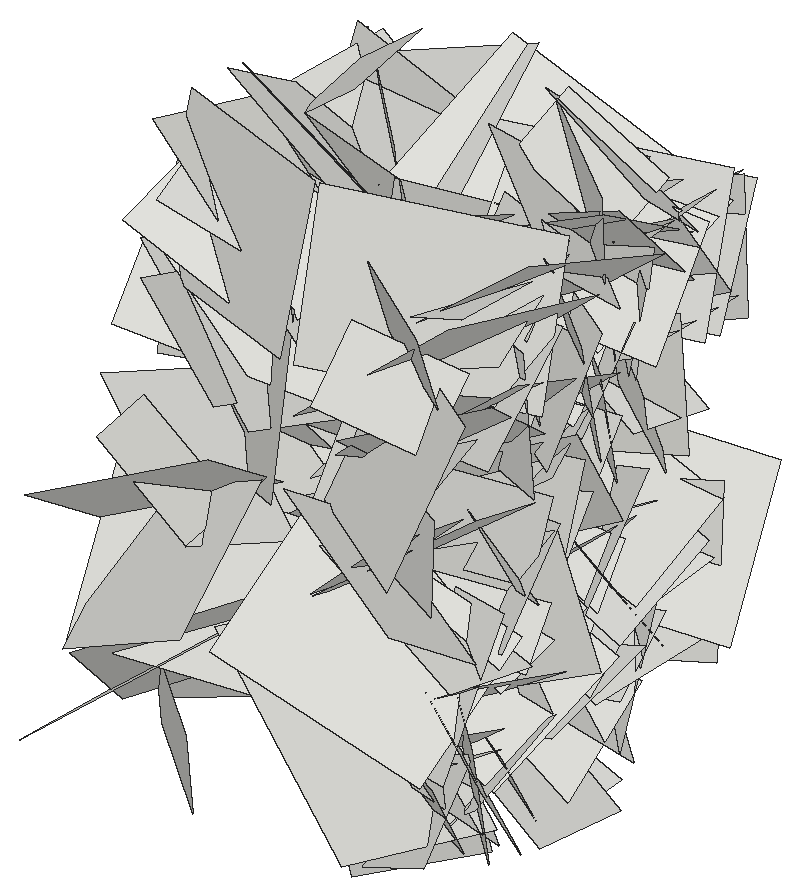
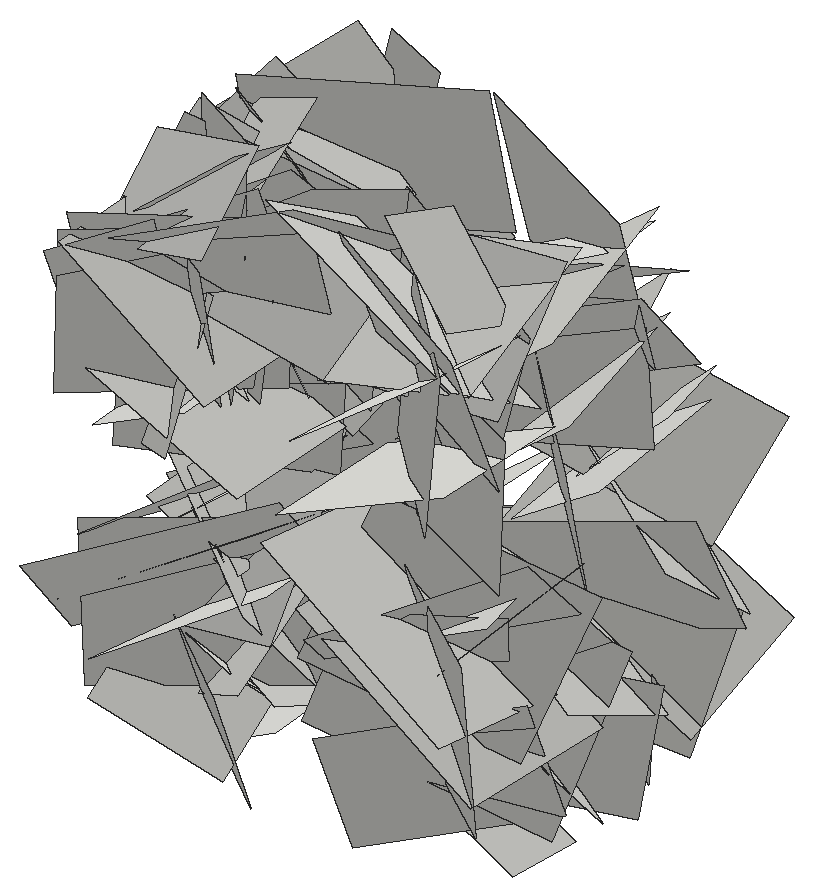
# SketchUp Ruby script. Lengths in inches.
U = 1.inch
M = Sketchup.active_model
def pt(a) = Geom::Point3d.new(a.map { |v| v * U })
def face(e, loops, mat)
  f = e.add_face(loops[0].map { |a| pt(a) })
  loops[1..].each { |l| e.add_face(l.map { |a| pt(a) }).erase! }
  f.material = f.back_material = mat if mat
  f
end
# faces: each face lists its corners as indices into pts; further lists are holes
def faces(e, pts, list, mat = nil) = list.each { |f| face(e, (f[0].is_a?(Array) ? f : [f]).map { |l| l.map { |i| pts[i] } }, mat) }
# xy, xz, yz: faces in a plane at the given z, y or x. An outline is a flat list of corners, or four numbers for a rectangle; further outlines are holes
def ring(l) = l.size == 4 ? [[l[0], l[1]], [l[2], l[1]], [l[2], l[3]], [l[0], l[3]]] : l.each_slice(2).to_a
def flat(e, list, mat, &to3) = list.each { |f| face(e, (f[0].is_a?(Array) ? f : [f]).map { |l| ring(l).map { |u, v| to3.(u, v) } }, mat) }
def xy(e, z, list, mat = nil) = flat(e, list, mat) { |x, y| [x, y, z] }
def xz(e, y, list, mat = nil) = flat(e, list, mat) { |x, z| [x, y, z] }
def yz(e, x, list, mat = nil) = flat(e, list, mat) { |y, z| [x, y, z] }
def lines(e, pts, list) = list.each { |a, b| e.add_line(pt(pts[a]), pt(pts[b])) }
# prism: a flat outline (further loops are holes) pulled along v
def prism(e, loops, v, mat = nil)
  f = face(e, loops, mat); d = Geom::Vector3d.new(v.map { |x| x * U })
  f.pushpull(f.normal.samedirection?(d) ? d.length : -d.length)
end
def box(e, o, s, mat = nil) = prism(e, [[o, [o[0] + s[0], o[1], o[2]], [o[0] + s[0], o[1] + s[1], o[2]], [o[0], o[1] + s[1], o[2]]]], [0, 0, s[2]], mat)
def at(x, y, z, deg = 0) = Geom::Transformation.translation(pt([x, y, z])) * Geom::Transformation.rotation(ORIGIN, Z_AXIS, deg.degrees)
def axes(o, x, y, z) = Geom::Transformation.new([*x, 0, *y, 0, *z, 0, *pt(o).to_a, 1])
def part(name) = M.definitions.add(name)
# library, detail: a bought-in or finely detailed component or shape, given as its bounding box
def library(name, o, s) = part(name).tap { |d| box(d.entities, o, s) }
def detail(e, o, s) = box(e.add_group.entities, o, s)
def put(e, d, t, mat = nil) = e.add_instance(d, t).tap { |i| i.material = mat if mat }
def group(e, t, mat = nil) = e.add_group.tap { |g| g.transformation = t; g.material = mat if mat }.entities
root = M.entities
c1 = part("Component\#6")
p = [[0.01,0,0],[0,3.24,4.54],[4.32,3.24,4.54],[4.33,0,0]]
faces(c1.entities,p,[[0,1,2,3]])
put(root,c1,axes([400.91,173.53,27.66],[0.08068,-0.97468,-0.75893],[0.01331,-0.75972,0.97695],[1.30935,0.06778,0.03684]))
put(root,c1,axes([414.68,173.53,27.66],[-0.08068,-0.97468,-0.75893],[-0.01331,-0.75972,0.97695],[-1.30935,0.06778,0.03684]))
put(root,c1,axes([400.91,172.42,21.79],[0.22827,-1.35966,0.24048],[-0.1567,0.21929,1.3722],[1.45519,0.2369,0.11004]))
put(root,c1,axes([414.68,172.42,21.79],[-0.22827,-1.35966,0.24048],[0.1567,0.21929,1.3722],[-1.45519,0.2369,0.11004]))
put(root,c1,axes([410.71,168.82,35.84],[0.04533,0.37689,0.51175],[-0.01637,0.51337,-0.3768],[0.67349,-0.01289,-0.04361]))
put(root,c1,axes([400.91,171.44,27.64],[0.05126,-0.8571,0.56567],[0.11133,0.56746,0.85083],[1.08285,-0.01777,-0.11425]))
put(root,c1,axes([414.68,171.44,27.64],[-0.05126,-0.8571,0.56567],[-0.11133,0.56746,0.85083],[-1.08285,-0.01777,-0.11425]))
put(root,c1,axes([414.68,167.34,31.77],[0.2501,0.51374,1.1242],[0.05799,1.13903,-0.532],[-1.3089,0.14863,0.19123]))
put(root,c1,axes([410.71,172.01,32.68],[0.01531,-0.04852,-0.71126],[0.05574,-0.70939,0.04946],[0.75363,0.05345,0.01079]))
put(root,c1,axes([404.88,172.58,29],[0.14706,-0.68518,0.03236],[0.10474,0.05263,0.69082],[-0.71951,-0.13238,0.10718]))
put(root,c1,axes([410.71,172.58,29],[-0.14706,-0.68518,0.03236],[-0.10474,0.05263,0.69082],[0.71951,-0.13238,0.10718]))
put(root,c1,axes([410.71,170.91,25.11],[0.00896,0.33986,-0.6335],[0.15678,-0.62081,-0.33108],[0.74574,0.12644,0.07722]))
put(root,c1,axes([410.71,171.42,39.46],[0.01769,0.21401,-0.61924],[0.03571,-0.6189,-0.21298],[0.69357,0.02641,0.02676]))
put(root,c1,axes([414.68,169.05,21.98],[-0.04882,0.58162,0.59704],[0.02934,0.59868,-0.58109],[-0.88303,-0.01226,-0.05232]))
put(root,c1,axes([410.71,173.67,32.24],[-0.05341,-0.65994,-0.37026],[-0.06447,-0.36634,0.66124],[0.79951,-0.07362,0.02859]))
put(root,c1,axes([404.88,170.73,19.61],[0.06378,-0.15247,0.68566],[0.07422,0.68605,0.14641],[-0.74085,0.05561,0.0737]))
put(root,c1,axes([410.71,170.73,19.61],[-0.06378,-0.15247,0.68566],[-0.07422,0.68605,0.14641],[0.74085,0.05561,0.0737]))
put(root,c1,axes([410.71,173.11,21.9],[-0.05319,-0.68826,0.19248],[-0.04456,0.19546,0.68797],[0.75624,-0.03689,0.05408]))
put(root,c1,axes([410.71,173.29,20.87],[0.09428,-0.62013,-0.08152],[0.03551,-0.0775,0.6261],[0.66205,0.09247,-0.02197]))
put(root,c1,axes([410.71,173.15,22.23],[0.01199,-0.5915,0.12784],[0.10227,0.12799,0.58366],[0.63327,-0.00947,-0.09668]))
put(root,c1,axes([414.68,174.01,26.46],[0.07872,-0.97306,0.24072],[-0.0738,0.23579,0.97461],[-1.05998,-0.08868,-0.04998]))
put(root,c1,axes([400.91,172.46,21.25],[0.14489,-0.73421,0.72244],[-0.08794,0.71856,0.74596],[1.0883,0.15581,-0.0359]))
put(root,c1,axes([414.68,172.46,21.25],[-0.14489,-0.73421,0.72244],[0.08794,0.71856,0.74596],[-1.0883,0.15581,-0.0359]))
put(root,c1,axes([400.91,169.91,24.28],[-0.0494,0.58776,1.07494],[0.25393,1.05932,-0.56884],[1.27358,-0.18841,0.15511]))
put(root,c1,axes([414.68,169.91,24.28],[0.0494,0.58776,1.07494],[-0.25393,1.05932,-0.56884],[-1.27358,-0.18841,0.15511]))
put(root,c1,axes([404.88,173.74,31.89],[0.15856,-0.67469,0.29232],[0.1064,0.31425,0.67394],[-0.77211,-0.09525,0.1529]))
put(root,c1,axes([410.71,173.74,31.89],[-0.15856,-0.67469,0.29232],[-0.1064,0.31425,0.67394],[0.77211,-0.09525,0.1529]))
put(root,c1,axes([414.68,172.13,35.78],[-0.07615,0.65901,-0.5201],[-0.04859,-0.52431,-0.658],[-0.88857,-0.02781,0.08055]))
put(root,c1,axes([400.91,171.47,32.36],[0.16942,0.96147,-0.31887],[-0.08969,-0.30901,-0.97416],[1.06999,-0.17814,-0.03117]))
put(root,c1,axes([414.68,171.47,32.36],[-0.16942,0.96147,-0.31887],[0.08969,-0.30901,-0.97416],[-1.06999,-0.17814,-0.03117]))
put(root,c1,axes([414.68,173.5,20.5],[0.29119,-0.77592,0.90535],[-0.00734,0.92801,0.79744],[-1.26387,-0.18415,0.20396]))
put(root,c1,axes([414.68,171.18,26.98],[0.09963,0.88743,-0.23237],[-0.05305,-0.22828,-0.89204],[-0.97094,0.10354,0.02489]))
put(root,c1,axes([414.68,170.16,39.2],[0.24703,1.2789,-0.21613],[0.13589,-0.24123,-1.28918],[-1.36812,0.20696,-0.16707]))
put(root,c1,axes([414.68,172,20.82],[0.19013,-0.4174,1.11707],[0.18593,1.12659,0.39279],[-1.25031,0.10406,0.22828]))
put(root,c1,axes([400.91,175.66,39.88],[-0.03914,-0.32872,-1.22009],[0.25418,-1.20026,0.31612],[1.31508,0.2222,-0.09741]))
put(root,c1,axes([414.68,175.66,39.88],[0.03914,-0.32872,-1.22009],[-0.25418,-1.20026,0.31612],[-1.31508,0.2222,-0.09741]))
put(root,c1,axes([410.71,171.52,27.71],[-0.03995,0.48298,0.66079],[-0.01207,0.66111,-0.48387],[0.8675,0.03144,0.0237]))
put(root,c1,axes([414.68,171.36,22.89],[-0.02535,0.88672,0.32576],[0.06435,0.32663,-0.88464],[-0.99927,-0.00146,-0.06523]))
put(root,c1,axes([414.68,175.14,30.45],[0.22771,0.17317,-1.07869],[-0.0194,-1.09862,-0.18001],[-1.15789,0.05246,-0.20912]))
put(root,c1,axes([414.68,174.95,31.63],[-0.12097,-0.07785,-0.70642],[-0.09105,-0.70871,0.09198],[-0.74781,0.09888,0.10307]))
put(root,c1,axes([414.68,176.52,27.27],[-0.06139,-0.83333,-0.30669],[0.14477,-0.31205,0.82208],[-0.93005,0.00643,0.1482]))
put(root,c1,axes([404.88,176.07,37.03],[0.15674,-0.62528,-0.09698],[-0.10666,-0.12156,0.63036],[-0.66219,-0.12843,-0.12449]))
put(root,c1,axes([410.71,176.07,37.03],[-0.15674,-0.62528,-0.09698],[0.10666,-0.12156,0.63036],[0.66219,-0.12843,-0.12449]))
put(root,c1,axes([400.91,172.47,36.95],[0.1233,0.89549,0.4145],[0.21728,0.38634,-0.89217],[1.02316,-0.18996,0.13951]))
put(root,c1,axes([414.68,172.47,36.95],[-0.1233,0.89549,0.4145],[-0.21728,0.38634,-0.89217],[-1.02316,-0.18996,0.13951]))
put(root,c1,axes([414.68,174.16,29.86],[-0.19319,0.59277,-0.26834],[-0.07097,-0.29428,-0.60458],[-0.68606,-0.13648,0.1381]))
put(root,c1,axes([414.68,171.95,33.74],[0.07102,0.70639,0.8167],[-0.11892,0.8184,-0.69866],[-1.13841,-0.04142,0.12393]))
put(root,c1,axes([400.91,171.95,33.74],[-0.07102,0.70639,0.8167],[0.11892,0.8184,-0.69866],[1.13841,-0.04142,0.12393]))
put(root,c1,axes([400.91,177.96,25.04],[0.10915,-1.1796,-0.55067],[0.03689,-0.5497,1.18402],[1.37942,0.10803,0.01191]))
put(root,c1,axes([414.68,177.96,25.04],[-0.10915,-1.1796,-0.55067],[-0.03689,-0.5497,1.18402],[-1.37942,0.10803,0.01191]))
put(root,c1,axes([400.91,178.09,32.9],[0.18757,-0.47698,-1.21124],[-0.23196,-1.21588,0.44684],[1.36024,-0.14157,0.24323]))
put(root,c1,axes([414.68,178.09,32.9],[-0.18757,-0.47698,-1.21124],[0.23196,-1.21588,0.44684],[-1.36024,-0.14157,0.24323]))
put(root,c1,axes([400.91,173.31,35.98],[-0.01252,1.07454,-0.37217],[-0.12805,-0.37127,-1.06811],[1.19858,-0.02844,-0.11799]))
put(root,c1,axes([414.68,173.31,35.98],[0.01252,1.07454,-0.37217],[0.12805,-0.37127,-1.06811],[-1.19858,-0.02844,-0.11799]))
put(root,c1,axes([414.68,176.41,32.2],[-0.11408,-0.0942,-0.79779],[-0.0272,-0.8041,0.09841],[-0.85109,0.03832,0.10379]))
put(root,c1,axes([414.68,172.625,27.43],[0.01975,0.58315,0.74345],[-0.01761,0.74368,-0.58292],[-1.00141,-0.00157,0.02491]))
put(root,c1,axes([400.91,174.78,20.26],[0.10048,-0.39109,0.79293],[0.10042,0.79738,0.38196],[0.93179,-0.04376,-0.12667]))
put(root,c1,axes([414.68,174.78,20.26],[-0.10048,-0.39109,0.79293],[-0.10042,0.79738,0.38196],[-0.93179,-0.04376,-0.12667]))
put(root,c1,axes([410.71,174.375,32.02],[-0.18574,0.64681,-0.5499],[-0.00393,-0.56207,-0.65994],[0.8999,0.13105,-0.11638]))
put(root,c1,axes([400.91,174.06,31.875],[0.08593,-0.00736,1.08266],[0.18405,1.07173,-0.00571],[1.1328,-0.17357,-0.0812]))
put(root,c1,axes([414.68,174.06,31.875],[-0.08593,-0.00736,1.08266],[-0.18405,1.07173,-0.00571],[-1.1328,-0.17357,-0.0812]))
put(root,c1,axes([414.68,176.05,33.17],[-0.01986,0.50916,-0.88553],[0.06176,-0.8837,-0.50934],[-1.08099,-0.05984,-0.01283]))
put(root,c1,axes([414.68,178.05,19.9375],[0.14578,-1.0409,0.22357],[0.02192,0.228,1.04879],[-1.1283,-0.13006,0.04926]))
put(root,c1,axes([410.71,177.7,39.03],[-0.08239,-0.33737,-0.64844],[0.10668,-0.65083,0.32654],[0.76743,0.05425,-0.11501]))
put(root,c1,axes([410.71,173.36,27.66],[-0.12062,0.63946,0.63128],[-0.06443,0.62939,-0.6485],[0.9503,0.12384,0.03616]))
put(root,c1,axes([400.91,173.84,39.64],[-0.13369,1.27699,-0.41872],[-0.11509,-0.42887,-1.27523],[1.41986,0.08547,-0.14279]))
put(root,c1,axes([414.68,173.84,39.64],[0.13369,1.27699,-0.41872],[0.11509,-0.42887,-1.27523],[-1.41986,0.08547,-0.14279]))
put(root,c1,axes([400.91,179.04,23.77],[0.11323,-0.75693,-0.7774],[0.09292,-0.77258,0.76428],[1.14637,0.13739,0.01483]))
put(root,c1,axes([414.68,179.04,23.77],[-0.11323,-0.75693,-0.7774],[-0.09292,-0.77258,0.76428],[-1.14637,0.13739,0.01483]))
put(root,c1,axes([414.68,174.875,32.24],[-0.12053,0.70886,0.38052],[0.08644,0.39248,-0.70676],[-0.84842,-0.06072,-0.12606]))
put(root,c1,axes([410.71,178.15,33.23],[0.08938,-0.00525,-0.60269],[-0.06829,-0.60515,-0.00374],[0.63521,-0.06432,0.0844]))
put(root,c1,axes([414.68,174.67,32.54],[0.17055,0.3665,0.95024],[0.03456,0.95968,-0.37566],[-1.07902,0.08867,0.13816]))
put(root,c1,axes([414.68,174.9,23.69],[0.06803,0.90477,0.33383],[-0.16872,0.33992,-0.89067],[-1.00823,0.00417,0.17157]))
put(root,c1,axes([410.71,175.43,34.87],[-0.0411,0.62613,0.35799],[-0.03637,0.3565,-0.62724],[0.76365,0.05068,-0.01061]))
put(root,c1,axes([414.68,178.01,36.42],[-0.04909,-0.68925,0.58112],[0.09024,0.57594,0.68989],[-0.95135,0.0902,0.03545]))
put(root,c1,axes([404.88,176.44,21.6],[0.04345,0.60879,-0.00304],[-0.10651,0.00376,-0.60183],[-0.63647,0.04093,0.10051]))
put(root,c1,axes([410.71,176.44,21.6],[-0.04345,0.60879,-0.00304],[0.10651,0.00376,-0.60183],[0.63647,0.04093,0.10051]))
put(root,c1,axes([404.88,180.42,25.12],[0.17902,-0.88337,-0.09354],[0.21931,-0.05348,0.8786],[-0.91571,-0.1855,0.19214]))
put(root,c1,axes([410.71,180.42,25.12],[-0.17902,-0.88337,-0.09354],[-0.21931,-0.05348,0.8786],[0.91571,-0.1855,0.19214]))
put(root,c1,axes([414.68,177.13,31.79],[0.078,-0.30439,1.03044],[0.07955,1.03178,0.29943],[-1.13614,0.05135,0.09171]))
put(root,c1,axes([400.91,179.625,37.91],[0.28026,0.12179,-1.29213],[0.26115,-1.29941,-0.07206],[1.35072,0.22596,0.28204]))
put(root,c1,axes([414.68,179.625,37.91],[-0.28026,0.12179,-1.29213],[-0.26115,-1.29941,-0.07206],[-1.35072,0.22596,0.28204]))
put(root,c1,axes([400.91,178.68,21.25],[0.14964,-1.02559,0.91665],[-0.24358,0.89093,1.03221],[1.43757,0.25771,0.07948]))
put(root,c1,axes([414.68,178.68,21.25],[-0.14964,-1.02559,0.91665],[0.24358,0.89093,1.03221],[-1.43757,0.25771,0.07948]))
put(root,c1,axes([414.68,176.26,32.94],[-0.03084,0.60524,0.59943],[0.03406,0.60013,-0.60439],[-0.90231,0.00196,-0.0433]))
put(root,c1,axes([400.91,177.97,39.67],[-0.02985,0.75948,-0.84861],[0.27983,-0.8214,-0.74388],[1.17429,0.21504,0.15569]))
put(root,c1,axes([414.68,177.97,39.67],[0.02985,0.75948,-0.84861],[-0.27983,-0.8214,-0.74388],[-1.17429,0.21504,0.15569]))
put(root,c1,axes([414.68,182.1,27.04],[0.18817,-1.1788,-0.21223],[0.10509,-0.19936,1.19019],[-1.26526,-0.19187,0.06729]))
put(root,c1,axes([400.91,177.28,39.83],[0.04784,1.11638,-0.64936],[0.22797,-0.64718,-1.09769],[1.34988,0.06974,0.20839]))
put(root,c1,axes([414.68,177.28,39.83],[-0.04784,1.11638,-0.64936],[-0.22797,-0.64718,-1.09769],[-1.34988,0.06974,0.20839]))
put(root,c1,axes([410.71,175.72,36.8],[-0.15665,0.75943,0.7145],[-0.11122,0.70715,-0.77331],[1.09966,0.17971,0.02357]))
put(root,c1,axes([410.71,180.11,41],[-0.0874,0.13713,-0.78202],[-0.02965,-0.78624,-0.13492],[0.84107,-0.01347,-0.08602]))
put(root,c1,axes([414.68,177.89,30.77],[-0.05678,-0.11721,0.8526],[0.09083,0.84928,0.12214],[-0.90772,0.09231,-0.04111]))
put(root,c1,axes([400.91,175.96,26.52],[0.03553,0.82214,0.9074],[-0.07429,0.90754,-0.81968],[1.2958,0.02948,-0.07187]))
put(root,c1,axes([414.68,175.96,26.52],[-0.03553,0.82214,0.9074],[0.07429,0.90754,-0.81968],[-1.2958,0.02948,-0.07187]))
put(root,c1,axes([404.88,180.68,27.18],[0.06604,-0.60003,0.10008],[-0.10227,0.08959,0.59716],[-0.63666,-0.07663,-0.08554]))
put(root,c1,axes([410.71,180.68,27.18],[-0.06604,-0.60003,0.10008],[0.10227,0.08959,0.59716],[0.63666,-0.07663,-0.08554]))
put(root,c1,axes([414.68,182.31,23.94],[0.04872,-1.30982,0.04089],[-0.01644,0.04037,1.31055],[-1.38898,-0.04642,-0.01408]))
put(root,c1,axes([400.91,182.31,23.94],[-0.04872,-1.30982,0.04089],[0.01644,0.04037,1.31055],[1.38898,-0.04642,-0.01408]))
put(root,c1,axes([400.91,180.07,24.39],[-0.06666,-0.76105,0.92501],[0.21989,0.90537,0.75899],[1.25053,-0.19976,-0.08415]))
put(root,c1,axes([414.68,180.07,24.39],[0.06666,-0.76105,0.92501],[-0.21989,0.90537,0.75899],[-1.25053,-0.19976,-0.08415]))
put(root,c1,axes([400.91,180.75,35.09],[-0.01445,0.08276,-1.11066],[0.1396,-1.10283,-0.0838],[1.17228,0.13235,-0.00371]))
put(root,c1,axes([414.68,180.75,35.09],[0.01445,0.08276,-1.11066],[-0.1396,-1.10283,-0.0838],[-1.17228,0.13235,-0.00371]))
put(root,c1,axes([414.68,177.99,23.55],[-0.04107,0.5427,0.4395],[-0.20397,0.41484,-0.52921],[-0.71159,-0.15024,0.12632]))
put(root,c1,axes([414.68,182.77,28.15],[0.11013,-1.0722,-0.31704],[0.03816,-0.31503,1.07721],[-1.18456,-0.10983,0.00522]))
put(root,c1,axes([404.88,178.13,40.15],[0.04908,0.64392,0.19174],[0.08573,0.18545,-0.64234],[-0.70699,0.06719,-0.06458]))
put(root,c1,axes([410.71,178.13,40.15],[-0.04908,0.64392,0.19174],[-0.08573,0.18545,-0.64234],[0.70699,0.06719,-0.06458]))
put(root,c1,axes([404.88,181.39,28.46],[0.11732,-0.15238,-0.58962],[-0.01785,-0.59981,0.15186],[-0.64528,-0.01111,-0.1114]))
put(root,c1,axes([410.71,181.39,28.46],[-0.11732,-0.15238,-0.58962],[0.01785,-0.59981,0.15186],[0.64528,-0.01111,-0.1114]))
put(root,c1,axes([400.91,183.19,37.72],[0.19709,-1.17807,-0.70591],[0.26547,-0.67132,1.18631],[1.43137,0.28672,-0.12282]))
put(root,c1,axes([414.68,183.19,37.72],[-0.19709,-1.17807,-0.70591],[-0.26547,-0.67132,1.18631],[-1.43137,0.28672,-0.12282]))
put(root,c1,axes([400.91,182.77,28.7],[-0.0358,-0.11408,-1.31406],[-0.04325,-1.31377,0.1151],[1.39747,-0.04358,-0.0301]))
put(root,c1,axes([414.68,182.77,28.7],[0.0358,-0.11408,-1.31406],[0.04325,-1.31377,0.1151],[-1.39747,-0.04358,-0.0301]))
put(root,c1,axes([414.68,178.01,21.81],[-0.00864,0.40014,0.99077],[0.02339,0.99065,-0.39991],[-1.13239,0.01741,-0.01582]))
put(root,c1,axes([400.91,178.01,21.81],[0.00864,0.40014,0.99077],[-0.02339,0.99065,-0.39991],[1.13239,0.01741,-0.01582]))
put(root,c1,axes([410.71,180.66,33.34],[-0.08177,-0.45253,0.73357],[0.03972,0.73405,0.45677],[0.91278,-0.07248,0.04584]))
put(root,c1,axes([414.68,183.77,26.5],[-0.0762,-1.33255,-0.21023],[-0.04546,-0.20817,1.33413],[-1.42926,0.07766,-0.03122]))
put(root,c1,axes([400.91,183.77,26.5],[0.0762,-1.33255,-0.21023],[0.04546,-0.20817,1.33413],[1.42926,0.07766,-0.03122]))
put(root,c1,axes([410.71,182.27,37.76],[-0.22679,0.05489,-0.89691],[-0.06736,-0.9206,-0.04118],[0.95012,-0.05216,-0.217]))
put(root,c1,axes([414.68,182.09,31.375],[-0.0562,-0.72005,0.10613],[-0.07977,0.11126,0.71729],[-0.76737,0.04117,-0.08234]))
put(root,c1,axes([400.91,183.25,38.77],[-0.07927,-0.40868,-1.12281],[0.1988,-1.11508,0.39337],[1.25087,0.15132,-0.13368]))
put(root,c1,axes([414.68,183.25,38.77],[0.07927,-0.40868,-1.12281],[-0.1988,-1.11508,0.39337],[-1.25087,0.15132,-0.13368]))
put(root,c1,axes([414.68,180.04,24.28],[-0.15161,0.71603,-0.23582],[-0.04269,-0.24694,-0.72538],[-0.79796,-0.12284,0.08362]))
put(root,c1,axes([410.71,181.67,36.78],[-0.05967,0.56874,-0.94691],[-0.29528,-0.9248,-0.5389],[1.13301,-0.21107,-0.19031]))
put(root,c1,axes([400.91,178.49,34.59],[0.00763,1.14917,-0.03145],[0.21412,-0.03223,-1.13128],[1.19962,-0.00155,0.20212]))
put(root,c1,axes([414.68,178.49,34.59],[-0.00763,1.14917,-0.03145],[-0.21412,-0.03223,-1.13128],[-1.19962,-0.00155,0.20212]))
put(root,c1,axes([414.68,181.8125,37.17],[0.0246,-0.63961,0.56311],[-0.17949,0.54862,0.63013],[-0.88529,-0.129,-0.11211]))
put(root,c1,axes([414.68,184.3,37.98],[0.01849,-0.42221,-1.00939],[0.24573,-0.98518,0.41609],[-1.13346,-0.22047,0.07374]))
put(root,c1,axes([414.68,185.38,28.27],[0.28552,-0.8956,-0.93898],[0.07116,-0.9481,0.92355],[-1.37362,-0.23528,-0.14733]))
put(root,c1,axes([400.91,183.67,38.38],[0.04708,0.10578,-1.15378],[-0.2342,-1.13267,-0.11235],[1.2056,-0.22416,0.02323]))
put(root,c1,axes([414.68,183.67,38.38],[-0.04708,0.10578,-1.15378],[0.2342,-1.13267,-0.11235],[-1.2056,-0.22416,0.02323]))
put(root,c1,axes([400.91,179.35,38.14],[0.07028,1.07405,0.02302],[-0.04111,0.02544,-1.07534],[1.13802,-0.06541,-0.04027]))
put(root,c1,axes([414.68,179.35,38.14],[-0.07028,1.07405,0.02302],[0.04111,0.02544,-1.07534],[-1.13802,-0.06541,-0.04027]))
